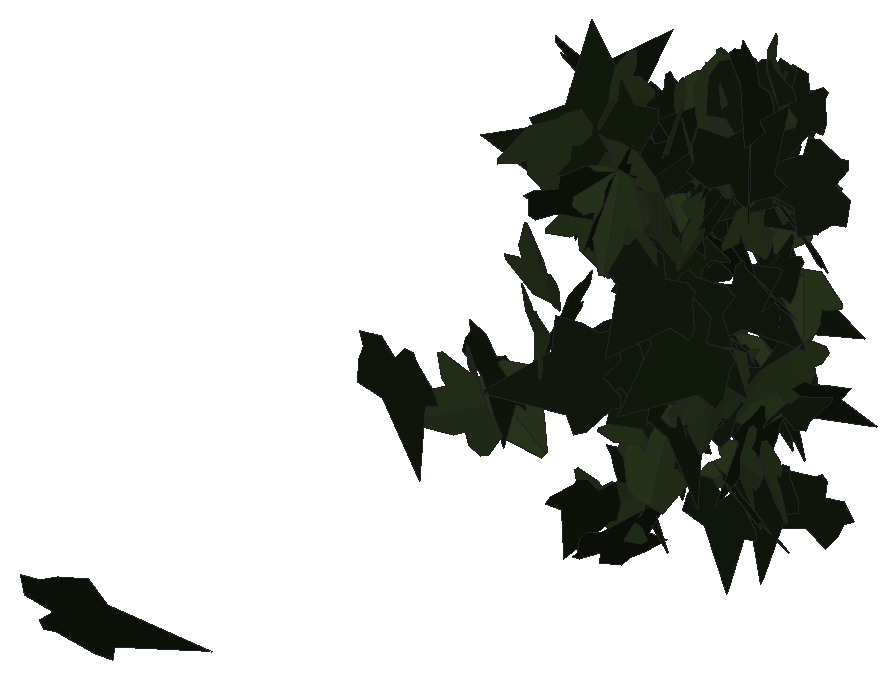
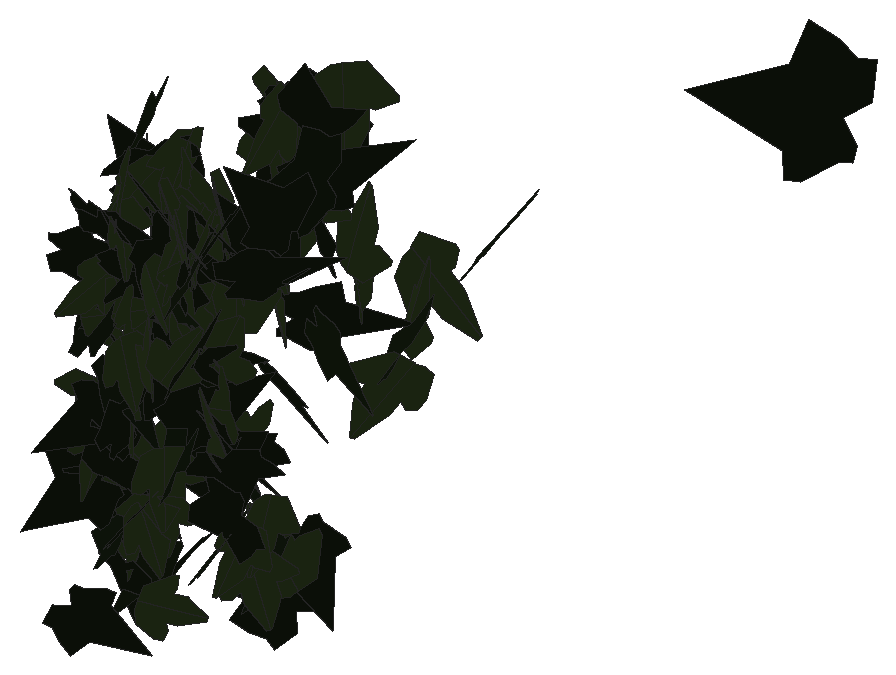
# SketchUp Ruby script. Lengths in inches.
U = 1.inch
M = Sketchup.active_model
def pt(a) = Geom::Point3d.new(a.map { |v| v * U })
def face(e, loops, mat)
  f = e.add_face(loops[0].map { |a| pt(a) })
  loops[1..].each { |l| e.add_face(l.map { |a| pt(a) }).erase! }
  f.material = f.back_material = mat if mat
  f
end
# faces: each face lists its corners as indices into pts; further lists are holes
def faces(e, pts, list, mat = nil) = list.each { |f| face(e, (f[0].is_a?(Array) ? f : [f]).map { |l| l.map { |i| pts[i] } }, mat) }
# xy, xz, yz: faces in a plane at the given z, y or x. An outline is a flat list of corners, or four numbers for a rectangle; further outlines are holes
def ring(l) = l.size == 4 ? [[l[0], l[1]], [l[2], l[1]], [l[2], l[3]], [l[0], l[3]]] : l.each_slice(2).to_a
def flat(e, list, mat, &to3) = list.each { |f| face(e, (f[0].is_a?(Array) ? f : [f]).map { |l| ring(l).map { |u, v| to3.(u, v) } }, mat) }
def xy(e, z, list, mat = nil) = flat(e, list, mat) { |x, y| [x, y, z] }
def xz(e, y, list, mat = nil) = flat(e, list, mat) { |x, z| [x, y, z] }
def yz(e, x, list, mat = nil) = flat(e, list, mat) { |y, z| [x, y, z] }
def lines(e, pts, list) = list.each { |a, b| e.add_line(pt(pts[a]), pt(pts[b])) }
# prism: a flat outline (further loops are holes) pulled along v
def prism(e, loops, v, mat = nil)
  f = face(e, loops, mat); d = Geom::Vector3d.new(v.map { |x| x * U })
  f.pushpull(f.normal.samedirection?(d) ? d.length : -d.length)
end
def box(e, o, s, mat = nil) = prism(e, [[o, [o[0] + s[0], o[1], o[2]], [o[0] + s[0], o[1] + s[1], o[2]], [o[0], o[1] + s[1], o[2]]]], [0, 0, s[2]], mat)
def at(x, y, z, deg = 0) = Geom::Transformation.translation(pt([x, y, z])) * Geom::Transformation.rotation(ORIGIN, Z_AXIS, deg.degrees)
def axes(o, x, y, z) = Geom::Transformation.new([*x, 0, *y, 0, *z, 0, *pt(o).to_a, 1])
def part(name) = M.definitions.add(name)
# library, detail: a bought-in or finely detailed component or shape, given as its bounding box
def library(name, o, s) = part(name).tap { |d| box(d.entities, o, s) }
def detail(e, o, s) = box(e.add_group.entities, o, s)
def put(e, d, t, mat = nil) = e.add_instance(d, t).tap { |i| i.material = mat if mat }
def group(e, t, mat = nil) = e.add_group.tap { |g| g.transformation = t; g.material = mat if mat }.entities
root = M.entities
M.materials.add("efeu1").color = [18, 25, 13]
M.materials.add("efeu2").color = [43, 57, 29]
c1 = part("ivyleaf_9")
p = [[1.54,2.16,1.25],[1.36,2.04,1.19],[-0.21,0.99,0.68],[-0.71,1.11,0.82],[-0.85,0.86,0.67],[-0.8,0.17,0.21],
  [-0.9,-0.01,0.1],[-0.67,-0.16,-0.02],[-0.08,-0.08,-0.05],[-0.03,-0.6,-0.4],[0.65,-0.88,-0.66],[0.83,-0.6,-0.49],
  [1.29,-0.42,-0.43],[1.8125,-0.07,-0.26],[1.21,0.44,0.15]]
faces(c1.entities,p,[[0,1,2,3,4,5,6,7,8,9,10,11,12,13,14]],"efeu1")
c2 = part("ivyleaf_10")
p = [[0,0.5,-0.03],[-0.0625,2.02,-0.43],[-0.19,2.01,-0.46],[-0.54,1.05,-0.29],[-0.52,0.625,-0.18],[-0.83,0.76,-0.28],
  [-1.16,0.64,-0.33],[-1.15,0.33,-0.24],[-0.77,-0.39,0.02],[-0.3,-0.51,0.16],[0.04,-0.48,0.23],[-0.02,2.01,-0.4375],
  [-0.06,2.01,-0.43],[0.04,-0.49,0.23],[0.67,-0.49,0.14],[1.38,0.36,-0.2],[1.375,0.51,-0.24],[0.81,0.65,-0.19],
  [0.62,0.59,-0.15],[0.6,1.09,-0.28],[0.5,1.23,-0.31]]
faces(c2.entities,p,[[0,1,2,3,4,5,6,7,8,9,10],[11,12,0,13,14,15,16,17,18,19,20]],"efeu2")
put(root,c1,axes([505.94,113.86,177.14],[0.83474,-0.23817,0.93657],[0.98295,-0.0561,-0.82782],[0.21424,1.18542,0.14899]))
put(root,c1,axes([506.5625,125.4,178.86],[0.28164,-0.90648,0.15572],[0.0611,-0.13951,-0.98084],[0.99038,0.26639,0.01622]))
put(root,c2,axes([508.16,126.32,177.84],[-0.52117,-0.00266,0.90213],[-0.92996,-0.11852,-0.49857],[0.11325,-0.98553,0.05752]))
put(root,c2,axes([507.5,127.53,176.95],[-0.70556,0.57097,-0.00424],[-0.01322,-0.0078,0.90224],[0.61653,0.65327,0.01448]))
put(root,c1,axes([506.6,129.04,177.36],[0.18304,-0.71685,0.45373],[0.11949,-0.42211,-0.76602],[0.8984,0.20219,0.00944]))
put(root,c2,axes([507.73,129.04,178.43],[-0.40077,0.20812,0.74842],[0.69247,-0.32706,0.44223],[0.41839,0.74068,-0.01502]))
put(root,c2,axes([509.96,129.14,182.94],[0.98889,-0.2625,0.12427],[0.12799,-0.02017,-0.99053],[0.28398,0.92318,0.01369]))
put(root,c1,axes([509.17,129.58,177.56],[-0.59712,-0.20831,0.69348],[-0.67718,-0.22696,-0.61443],[0.33265,-0.83594,-0.00599]))
put(root,c2,axes([508.1875,129.17,183.86],[-0.4111,-0.86495,-0.08979],[0.01683,0.08745,-0.98256],[0.93864,-0.38039,-0.0217]))
put(root,c2,axes([507.81,129.25,179.62],[-0.84668,0.27498,-0.07489],[-0.07453,0.0208,0.86401],[0.2978,0.78699,0.00333]))
put(root,c2,axes([506.71,128.9,176.61],[0.39336,0.65574,0.55965],[0.266,0.47865,-0.77997],[-0.87667,0.43946,0.01446]))
put(root,c1,axes([508.72,128.85,182.68],[0.68116,0.67219,0.18803],[0.13172,0.13348,-0.95862],[-0.74014,0.64238,0.00244]))
put(root,c1,axes([510.23,130.62,180.03],[-0.45288,-0.69543,0.45021],[0.00427,-0.48803,-0.81138],[0.88468,-0.35364,0.23438]))
put(root,c1,axes([509.68,129.22,182.49],[-0.24621,0.31706,-0.86209],[-0.65238,0.57158,0.40015],[0.70222,0.64218,0.06948]))
put(root,c1,axes([511.15,130.95,178.52],[-0.57191,-0.59736,0.48023],[-0.25599,-0.40397,-0.8262],[0.7742,-0.57485,0.08157]))
put(root,c1,axes([507.75,130.93,182.16],[-0.20073,-0.05564,0.88155],[-0.83171,-0.35518,-0.19985],[0.38721,-0.79177,0.02771]))
put(root,c2,axes([508.63,130.43,181.375],[-0.67668,-0.66856,-0.08114],[0.08426,0.03374,-0.95227],[0.72204,-0.63049,0.03508]))
put(root,c2,axes([509.2,130.6,179.26],[0.46101,-0.7696,-0.06224],[-0.02012,0.05809,-0.91517],[0.83343,0.4271,0.01233]))
put(root,c1,axes([508.61,130.52,183.05],[-0.83244,-0.39889,0.41707],[0.38337,0.18661,0.90259],[-0.47561,0.84859,-0.00244]))
put(root,c1,axes([507.54,130.84,178.35],[-0.62529,0.44203,-0.31225],[0.232,-0.21281,-0.75664],[-0.52841,-0.6165,0.0373]))
put(root,c2,axes([508.76,130.68,182.82],[-1.01284,0.11567,-0.0065],[0.00574,-0.00802,-0.98269],[-0.12498,-0.9378,0.00761]))
put(root,c2,axes([509.23,130.84,180.86],[-0.74753,0.22428,0.53438],[-0.57388,-0.0021,-0.74347],[-0.1931,-0.86203,0.14085]))
put(root,c1,axes([510.37,130.99,179.32],[0.20092,-0.62334,-0.65989],[0.05352,0.6545,-0.65358],[0.95914,0.09405,0.1747]))
put(root,c2,axes([509.89,130.67,174.51],[0.13358,0.69526,-0.59978],[0.0348,0.60182,0.70538],[0.91756,-0.12405,0.06056]))
put(root,c1,axes([507.72,130.79,180.97],[-0.07012,0.17396,0.79838],[-0.30824,0.71266,-0.19305],[-0.79225,-0.29267,0.00445]))
put(root,c2,axes([511.04,131.45,177.86],[-0.57455,-0.66112,0.30091],[-0.1715,-0.2434,-0.88207],[0.76029,-0.55451,0.02843]))
put(root,c1,axes([508.46,131.53,177.28],[-0.79933,0.10661,-0.18091],[0.18302,-0.04324,-0.77744],[-0.1227,-0.75906,0.01887]))
put(root,c1,axes([507.68,131.47,173.16],[0.18297,0.53427,-0.53523],[-0.15745,-0.49362,-0.58285],[-0.78554,0.22338,-0.00784]))
put(root,c2,axes([508.39,131.21,183.96],[-0.03575,-0.40449,-0.85205],[0.08605,0.81542,-0.42204],[0.98303,-0.08609,0.00596]))
put(root,c1,axes([509.4,132.24,175.54],[0.26098,-0.74133,0.25178],[0.08695,-0.22838,-0.81089],[0.83775,0.25465,0.00573]))
put(root,c2,axes([507.57,131.92,172.45],[-0.64545,-0.17287,0.61518],[0.64172,0.05694,0.64165],[-0.17655,0.83894,0.08321]))
put(root,c2,axes([510.73,132.02,176.82],[-0.13755,-0.93242,0.07887],[-0.01473,-0.07755,-0.94251],[0.93564,-0.1383,-0.00324]))
put(root,c2,axes([511.01,131.46,177.77],[0.29406,-0.53723,-0.7019],[0.07126,0.71862,-0.56723],[0.9289,0.11494,0.26571]))
put(root,c1,axes([507.59,131.81,171.48],[0.53296,0.65943,0.02273],[-0.01729,-0.01531,0.85657],[0.71236,-0.49372,0.00379]))
put(root,c2,axes([508.2,132.58,180.04],[0.03662,-0.05263,0.75525],[0.39549,-0.62712,-0.06505],[0.67967,0.36775,-0.00284]))
put(root,c1,axes([506.125,132.51,183.54],[0.77972,-0.36529,0.31679],[0.28121,-0.14641,-0.86095],[0.39334,0.82878,-0.01247]))
put(root,c1,axes([509.55,132.64,175.87],[-0.71855,0.34879,0.31705],[-0.31343,0.10202,-0.78009],[-0.38996,-0.7247,0.04278]))
put(root,c1,axes([508.61,132.85,175.78],[-0.26023,-0.77132,-0.42107],[0.17362,0.38536,-0.81321],[0.86144,-0.31067,0.0367]))
put(root,c1,axes([509.33,132.59,175.04],[0.15278,0.10159,0.81469],[-0.71231,0.45313,0.06276],[-0.46946,-0.65447,0.16991]))
put(root,c2,axes([508.24,132.95,179.56],[-0.86715,0.0751,0.31552],[0.30163,-0.14434,0.86332],[0.11923,0.91141,0.11072]))
put(root,c1,axes([507.32,133.02,173.07],[0.45816,-0.5812,0.14001],[0.07035,-0.11908,-0.74812],[0.64046,0.42884,-0.01799]))
put(root,c1,axes([508.95,132.71,176.18],[-0.56695,0.63286,-0.04701],[0.04146,-0.02687,-0.85504],[-0.68397,-0.52621,-0.01287]))
put(root,c1,axes([509.22,133.27,176.37],[0.78785,-0.41477,-0.07351],[0.06445,-0.03804,0.87272],[-0.44982,-0.73192,-0.00371]))
put(root,c1,axes([510.51,132.84,181.8125],[-0.38535,-0.05657,0.72827],[0.75754,-0.07292,0.36557],[0.04273,0.78253,0.08671]))
put(root,c1,axes([510.51,133.43,182.48],[-0.09337,-0.04144,-0.79101],[0.78313,-0.23891,-0.07218],[-0.25194,-0.72725,0.06879]))
put(root,c1,axes([507.54,133.03,180.92],[-0.29681,-0.10776,0.86627],[0.85717,-0.20915,0.26767],[0.16522,0.8915,0.16751]))
put(root,c2,axes([510.33,133.53,174.1],[0.10339,-0.1058,-0.77136],[0.49702,-0.58173,0.14808],[-0.63849,-0.46996,-0.00964]))
put(root,c1,axes([507.67,133.62,180.87],[-0.41267,-0.00958,0.75701],[-0.72977,-0.30114,-0.37302],[0.29246,-0.76495,0.13737]))
put(root,c1,axes([509.59,133.64,172.65],[0.08013,-0.73845,0.17229],[0.04555,-0.16217,-0.77141],[0.81608,0.08156,0.02614]))
put(root,c1,axes([510.42,133.93,183.75],[0.0742,-0.54991,0.6777],[0.07063,-0.67413,-0.55474],[0.86988,0.10165,-0.01276]))
put(root,c2,axes([508.52,133.36,182.78],[0.39022,-0.7038,-0.26722],[-0.10957,0.23667,-0.82258],[0.80172,0.37491,0.01765]))
put(root,c1,axes([508.95,133.72,182.12],[-0.85663,0.05652,-0.19843],[0.20266,-0.04849,-0.82623],[-0.07152,-0.81436,0.03543]))
put(root,c1,axes([509.4,133.75,175.42],[-0.88225,-0.00069,0.01399],[-0.01452,-0.00763,-0.84954],[0.00088,-0.81697,0.00792]))
put(root,c1,axes([506.5,133.3125,182.53],[-0.07243,-0.20889,0.71233],[0.72784,0.21415,0.13655],[-0.26144,0.65405,0.1828]))
put(root,c2,axes([508.93,133.75,183.28],[0.69594,-0.20334,0.38103],[0.38306,-0.09316,-0.70255],[0.24096,0.73539,0.01636]))
put(root,c2,axes([507.22,133.81,173.54],[-0.57464,-0.43077,0.24116],[-0.17833,-0.16437,-0.71159],[0.49735,-0.55665,0.02349]))
put(root,c2,axes([509.45,133.4375,183.74],[-0.04415,0.79132,0.27924],[-0.08787,0.26377,-0.82137],[-0.89819,-0.0647,0.06663]))
put(root,c2,axes([508.9,133.7,182.19],[-0.83461,0.12141,-0.25732],[0.25613,-0.08233,-0.81236],[-0.15165,-0.80725,0.04415]))
put(root,c1,axes([507.76,133.85,182.6],[0.45081,-0.59639,-0.29772],[-0.17081,0.23871,-0.75704],[0.69374,0.44632,0.00707]))
put(root,c2,axes([506.74,133.75,175.14],[-0.12999,-0.67933,-0.27716],[0.18615,0.23599,-0.70659],[0.76582,-0.17267,0.12471]))
put(root,c1,axes([509.8,133.65,173.18],[0.76072,-0.17182,-0.27264],[-0.24665,0.16034,-0.74745],[0.23187,0.73428,0.09941]))
put(root,c2,axes([508.72,134.36,179.82],[0.07484,-0.56141,0.54544],[0.09325,-0.51756,-0.58805],[0.82447,0.1095,0.017]))
put(root,c1,axes([510.28,134.28,174.7],[-0.22547,0.24685,-0.69018],[0.39291,-0.55618,-0.33418],[-0.65605,-0.41793,0.03706]))
put(root,c1,axes([509.91,134.16,183.69],[-0.12848,-0.75221,-0.29134],[0.10338,0.27723,-0.76135],[0.8,-0.15663,0.0516]))
put(root,c2,axes([508.51,133.77,182.12],[-0.42115,0.69431,0.11009],[-0.06017,0.09012,-0.82816],[-0.75613,-0.39389,0.00458]))
put(root,c1,axes([508.8125,134.14,176.14],[0.21994,-0.74322,-0.33026],[-0.10023,0.31474,-0.77506],[0.8071,0.24162,-0.00626]))
put(root,c1,axes([508.02,134.53,179.14],[-0.53716,-0.60024,-0.09155],[0.1391,0.00676,-0.80476],[0.64026,-0.50506,0.09803]))
put(root,c2,axes([510.26,134.375,173.66],[-0.39318,0.35078,-0.54617],[0.39089,-0.38087,-0.52551],[-0.55895,-0.51311,0.01669]))
put(root,c1,axes([509.78,133.9,178.25],[0.00298,-0.2647,-0.73262],[0.15303,0.71854,-0.259],[0.76379,-0.14294,0.05475]))
put(root,c2,axes([510.16,133.95,175.1875],[-0.15741,-0.68372,0.48925],[0.11488,0.47559,0.70159],[-0.83285,0.19482,0.00431]))
put(root,c1,axes([508.13,134.46,177.42],[-0.78258,0.16383,-0.14702],[0.14659,-0.04065,-0.77256],[-0.18201,-0.73716,0.00993]))
put(root,c1,axes([509.17,134.29,180.45],[-0.65801,0.49767,-0.07882],[0.06436,-0.04685,-0.81816],[-0.53986,-0.61217,-0.00147]))
put(root,c1,axes([508.64,134.47,179.82],[-0.02698,-0.0287,-0.68719],[0.6946,0.15315,-0.0322],[0.16657,-0.64325,0.02299]))
put(root,c2,axes([507.77,134.32,179.05],[0.76981,0.16274,0.3275],[-0.33145,-0.07054,0.76037],[0.19156,-0.77605,-0.00044]))
put(root,c1,axes([508.46,134.62,181.75],[0.41022,-0.05187,-0.56176],[0.58273,-0.034,0.39799],[-0.06231,-0.65946,0.02367]))
put(root,c1,axes([510.14,134.7,172.96],[-0.57934,-0.14104,-0.55861],[0.54784,0.11038,-0.59604],[0.17836,-0.79719,0.0163]))
put(root,c1,axes([508.13,134.84,177.4375],[0.02148,0.0002,0.79719],[-0.78885,-0.23258,0.01977],[0.25111,-0.73066,-0.00608]))
put(root,c2,axes([508.62,134.6,182.49],[0.34062,-0.72726,-0.00598],[-0.00189,0.00572,-0.80307],[0.72728,0.34063,0.00072]))
put(root,c1,axes([508.87,134.6875,178.33],[0.53109,-0.35035,0.48893],[0.4188,-0.26587,-0.6279],[0.47494,0.62622,0.00695]))
put(root,c2,axes([509.88,134.16,183.05],[-0.14368,-0.49022,-0.63426],[0.38854,0.52103,-0.49072],[0.70117,-0.38917,0.14196]))
put(root,c1,axes([509.19,134.92,182],[-0.20284,0.29221,-0.65867],[0.36509,-0.53558,-0.36125],[-0.65891,-0.38671,0.0026]))
put(root,c2,axes([507.54,134.59,177.01],[0.5204,-0.60052,0.08039],[-0.02206,0.08262,0.79989],[-0.65355,-0.48097,0.03702]))
put(root,c2,axes([509.82,134.57,180.02],[-0.11681,-0.73215,-0.26513],[0.16077,0.233,-0.7616],[0.8217,-0.14966,0.11132]))
put(root,c1,axes([510.54,134.85,178.875],[-0.72615,0.13201,-0.20323],[0.20923,-0.02745,-0.71253],[-0.14522,-0.69964,-0.01039]))
put(root,c1,axes([509.2,134.3125,180.62],[0.04781,-0.06991,-0.82447],[0.26869,0.75541,-0.05483],[0.81642,-0.24452,0.06633]))
put(root,c1,axes([509.63,134.58,182.77],[-0.55515,0.42165,0.32907],[-0.26393,0.20099,-0.69143],[-0.50448,-0.56916,-0.00039]))
put(root,c1,axes([508.26,135.26,176.38],[0.56333,-0.24968,-0.50922],[0.46489,-0.20781,0.61618],[-0.32485,-0.73038,-0.00124]))
put(root,c2,axes([506.82,134.49,174.76],[-0.21331,-0.53067,-0.48237],[0.15703,0.45648,-0.57163],[0.69973,-0.26422,-0.01877]))
put(root,c1,axes([510.36,135.21,181.05],[-0.66517,-0.27252,0.21333],[-0.18773,-0.11353,-0.69965],[0.31696,-0.63916,0.03331]))
put(root,c2,axes([510.81,134.65,176.26],[-0.31487,-0.69452,-0.3284],[0.16253,0.28665,-0.76208],[0.75086,-0.35329,0.02725]))
put(root,c1,axes([506.9,135.13,177.05],[-0.47654,-0.55415,-0.24516],[0.15694,0.18839,-0.73086],[0.58529,-0.5017,-0.00364]))
put(root,c1,axes([508.48,135.22,180.64],[0.29035,-0.66519,0.02702],[0.01549,0.0338,0.74568],[-0.71879,-0.26797,0.02698]))
put(root,c1,axes([511.53,135.19,180.99],[-0.29054,-0.36184,-0.62774],[-0.41822,-0.46854,0.46363],[-0.59167,0.50886,-0.01947]))
put(root,c2,axes([508.97,134.6875,183.1],[0.30916,-0.34431,-0.51812],[-0.35278,0.37623,-0.46562],[0.55074,0.43428,-0.0074]))
put(root,c1,axes([510.51,134.67,174.99],[-0.66977,-0.08236,0.4732],[0.46854,0.06664,0.67477],[-0.10569,0.81735,-0.00733]))
put(root,c1,axes([508.28,135.03,178.7],[-0.08361,-0.66458,0.30944],[0.07713,0.29084,0.69494],[-0.78261,0.09966,0.03543]))
put(root,c2,axes([508.9,135.32,172.61],[-0.10542,-0.15586,0.6286],[-0.31049,-0.53179,-0.19091],[0.59837,-0.3034,0.01169]))
put(root,c2,axes([510.54,135.27,179.7],[-0.14487,-0.02874,-0.71071],[-0.70597,-0.19958,0.14218],[-0.21742,0.6672,0.01191]))
put(root,c1,axes([508.43,135.71,181.34],[-0.16966,-0.14497,0.77042],[-0.06007,-0.78354,-0.16066],[0.78164,-0.09168,0.15487]))
put(root,c2,axes([509.92,135.11,177.88],[0.59859,-0.46511,-0.21523],[-0.07664,0.23236,-0.74076],[0.54444,0.54409,0.13236]))
put(root,c1,axes([510.56,135.53,179.11],[0.47033,-0.52636,0.05741],[-0.02025,0.0561,0.71014],[-0.57122,-0.43538,0.0221]))
put(root,c2,axes([506.55,135.46,178.64],[0.25472,-0.1461,0.64694],[0.63231,-0.21621,-0.28368],[0.27645,0.62916,0.05274]))
put(root,c1,axes([509.95,135.27,178.48],[-0.39541,0.57459,-0.30149],[0.14514,-0.25791,-0.70816],[-0.67974,-0.38931,0.02417]))
put(root,c2,axes([508.24,135.57,179.14],[-0.29356,-0.31585,-0.42985],[-0.30768,-0.2998,0.43311],[-0.47005,0.39349,-0.01504]))
put(root,c2,axes([508.61,134.76,181.5625],[0.16742,-0.24231,0.79637],[-0.46991,0.643,0.29443],[-0.6871,-0.49879,-0.00731]))
put(root,c2,axes([510.0625,134.91,183.53],[-0.35857,0.37261,0.542],[-0.38307,0.38191,-0.51897],[-0.57619,-0.48578,0.00773]))
put(root,c1,axes([506.35,135.32,175.88],[0.13074,-0.17181,-0.73096],[0.65475,0.38931,0.0256],[0.36759,-0.63233,0.21437]))
put(root,c1,axes([506.6,135.4,175.26],[0.41275,-0.62654,-0.12931],[-0.05875,0.11611,-0.75014],[0.63705,0.41666,0.0146]))
put(root,c2,axes([508.68,135.74,178.85],[0.16123,-0.40579,-0.56306],[0.19796,-0.50943,0.44967],[-0.7034,-0.23638,-0.00251]))
put(root,c2,axes([510.47,135.43,177.86],[0.73518,0.19283,0.10718],[0.09835,0.04733,-0.75977],[-0.19748,0.74144,0.02063]))
put(root,c2,axes([508.47,135.4,176.5],[-0.40157,-0.63426,-0.04932],[0.01558,0.04651,-0.76453],[0.68673,-0.37194,-0.01149]))
put(root,c2,axes([509.67,135.43,182.62],[0.05875,-0.71034,-0.13607],[-0.012,0.13554,-0.71276],[0.72315,0.05996,-0.00078]))
put(root,c1,axes([510.72,135.06,175.14],[0.62077,0.30151,0.27518],[0.24669,0.13407,-0.67492],[-0.35615,0.6184,0.01215]))
put(root,c1,axes([510.41,135.73,182.74],[-0.6764,-0.07143,-0.30059],[0.31461,-0.00803,-0.65442],[0.06639,-0.68972,0.03875]))
put(root,c2,axes([508.52,135.54,175.45],[0.68834,0.32129,-0.02725],[-0.02409,-0.01397,-0.7423],[-0.34732,0.63774,-0.00253]))
put(root,c1,axes([510.01,135.82,182.61],[-0.69905,-0.20245,-0.08993],[0.0896,0.02441,-0.70531],[0.22023,-0.65256,0.00151]))
put(root,c2,axes([510.46,135.13,180.64],[-0.13803,-0.27074,-0.66229],[0.33899,0.55445,-0.31067],[0.66603,-0.33831,0.02087]))
put(root,c2,axes([509.41,135.69,179.25],[-0.1316,-0.69862,0.05535],[-0.01342,-0.0538,-0.7109],[0.70068,-0.13224,-0.00322]))
put(root,c2,axes([508.77,135.76,175.18],[-0.14589,-0.69145,0.12274],[-0.05113,-0.11093,-0.73225],[0.75584,-0.14097,-0.02584]))
put(root,c1,axes([509.3,135.93,174.66],[0.32457,-0.57675,0.28713],[0.15451,-0.23667,-0.67616],[0.67307,0.33245,0.01676]))
put(root,c1,axes([510.73,135.875,172.15],[-0.05372,0.03797,-0.69504],[-0.37128,-0.57647,-0.00745],[-0.62031,0.34175,0.06465]))
put(root,c1,axes([509.47,136.05,177.12],[-0.00311,0.08788,0.68584],[-0.36609,-0.56764,0.07713],[0.61825,-0.33568,0.04912]))
put(root,c2,axes([508.52,135.8,181.59],[0.18387,-0.68333,0.09055],[0.00857,-0.09144,-0.70747],[0.68925,0.18343,-0.01536]))
put(root,c1,axes([509.99,135.22,177.45],[0.04466,-0.00828,-0.77504],[0.17642,0.72833,0.00101],[0.78533,-0.16315,0.04385]))
put(root,c1,axes([508.96,135.77,175.22],[0.29914,-0.6481,-0.12268],[-0.01571,0.12192,-0.73214],[0.71127,0.27526,0.03542]))
